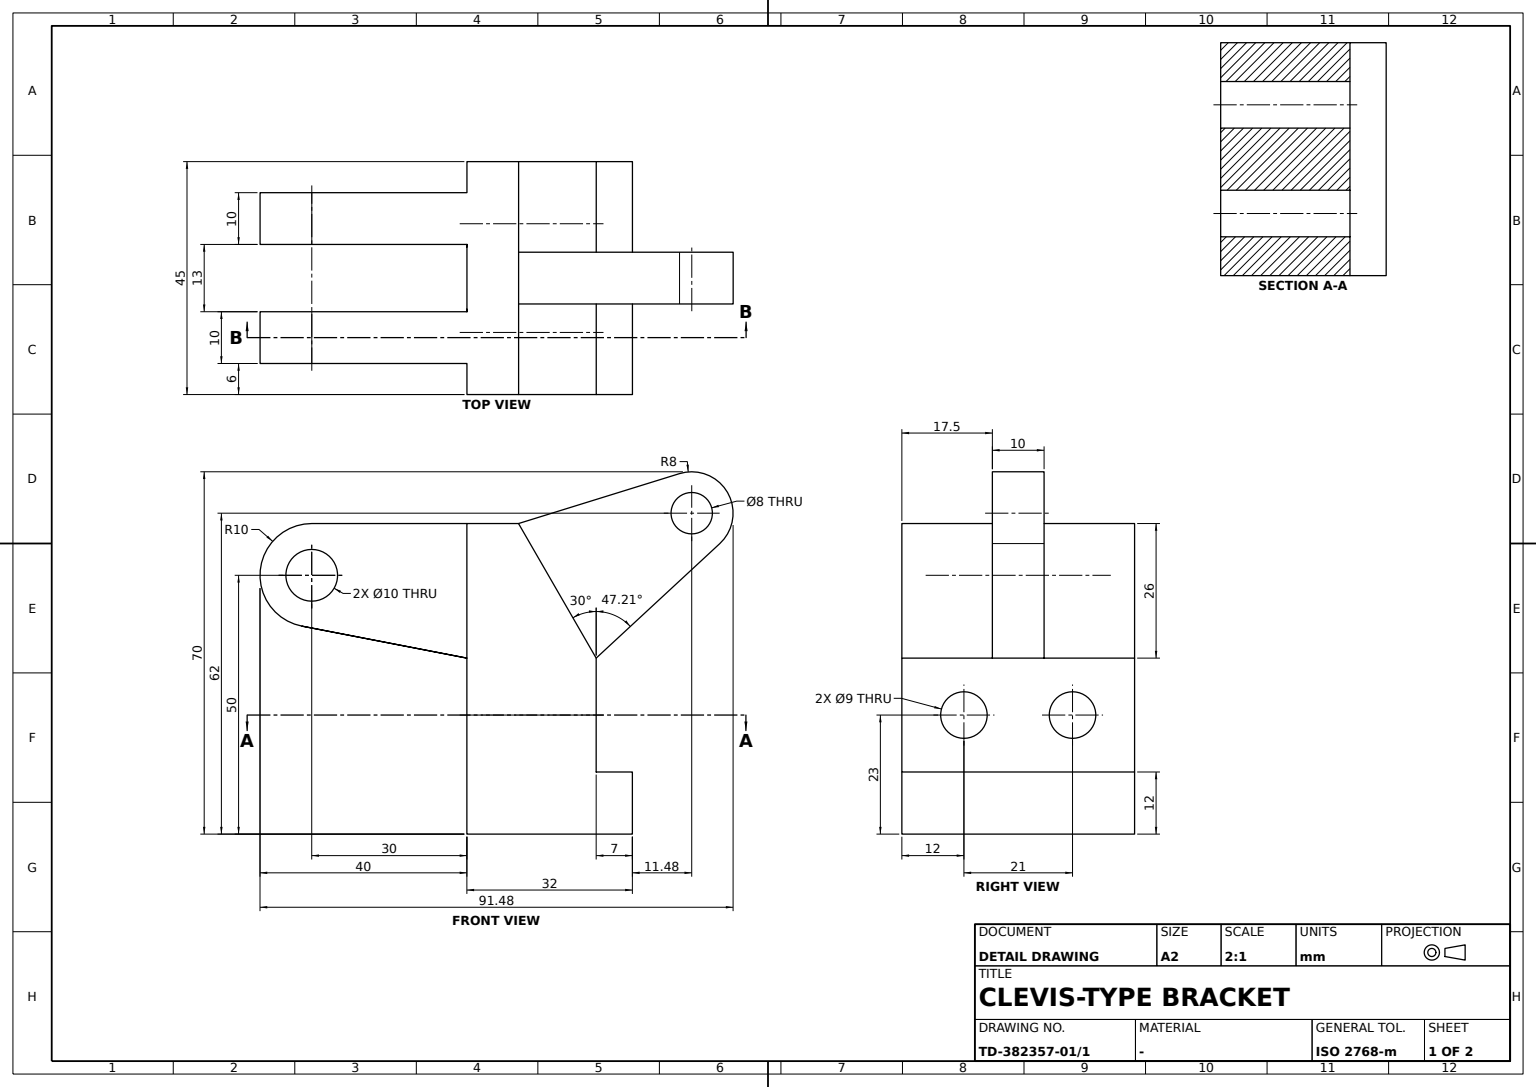
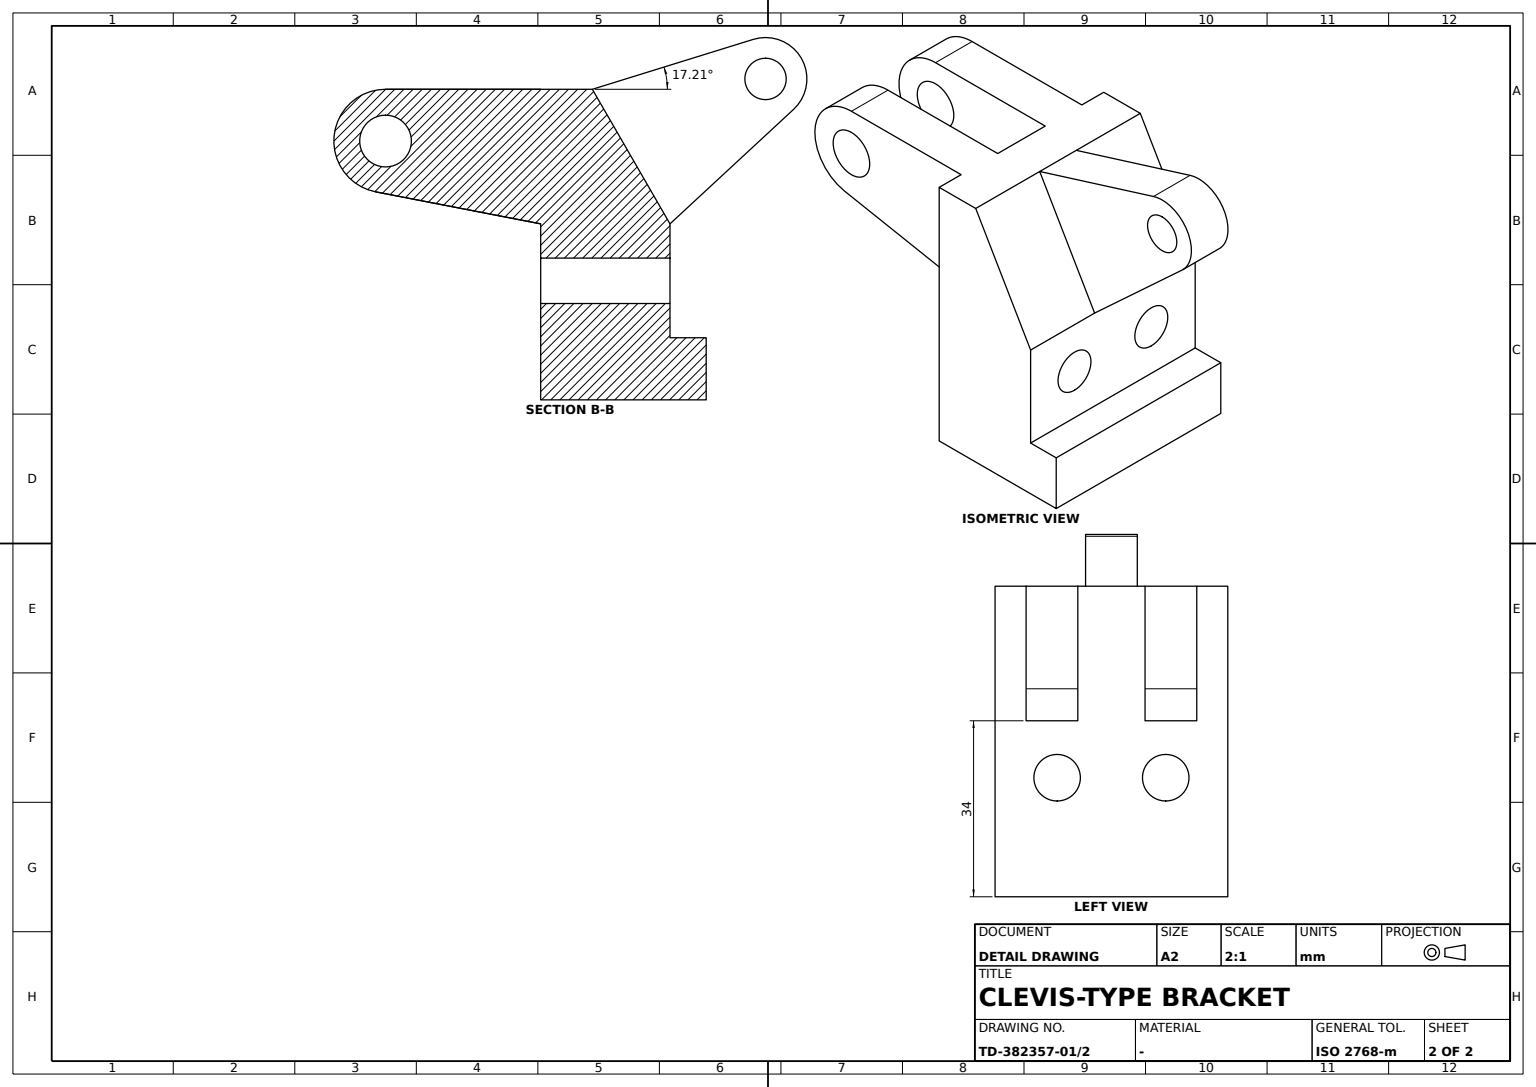
ISO-10303-21;
HEADER;
FILE_DESCRIPTION((''),'2;1');
FILE_NAME('','',(''),(''),'','','');
FILE_SCHEMA(('AUTOMOTIVE_DESIGN'));
ENDSEC;
DATA;
#1=APPLICATION_CONTEXT('');
#2=PRODUCT_CONTEXT('',#1,'mechanical');
#3=PRODUCT('','','',(#2));
#4=PRODUCT_DEFINITION_FORMATION('','',#3);
#5=PRODUCT_DEFINITION_CONTEXT('',#1,'design');
#6=PRODUCT_DEFINITION('','',#4,#5);
#7=PRODUCT_DEFINITION_SHAPE('','',#6);
#8=(LENGTH_UNIT()NAMED_UNIT(*)SI_UNIT(.MILLI.,.METRE.));
#9=(NAMED_UNIT(*)PLANE_ANGLE_UNIT()SI_UNIT($,.RADIAN.));
#10=(NAMED_UNIT(*)SI_UNIT($,.STERADIAN.)SOLID_ANGLE_UNIT());
#11=UNCERTAINTY_MEASURE_WITH_UNIT(LENGTH_MEASURE(0.005),#8,'distance_accuracy_value','');
#12=(GEOMETRIC_REPRESENTATION_CONTEXT(3)GLOBAL_UNCERTAINTY_ASSIGNED_CONTEXT((#11))GLOBAL_UNIT_ASSIGNED_CONTEXT((#8,#9,#10))REPRESENTATION_CONTEXT('',''));
#13=CARTESIAN_POINT('',(0.,22.5,0.));
#14=VERTEX_POINT('',#13);
#15=CARTESIAN_POINT('',(0.,22.5,12.));
#16=VERTEX_POINT('',#15);
#17=DIRECTION('',(0.,0.,1.));
#18=VECTOR('',#17,1000.);
#19=LINE('',#13,#18);
#20=EDGE_CURVE('',#14,#16,#19,.T.);
#21=ORIENTED_EDGE('',*,*,#20,.T.);
#22=CARTESIAN_POINT('',(0.,-22.5,12.));
#23=VERTEX_POINT('',#22);
#24=CARTESIAN_POINT('',(0.,0.,12.));
#25=DIRECTION('',(0.,1.,0.));
#26=VECTOR('',#25,1000.);
#27=LINE('',#24,#26);
#28=EDGE_CURVE('',#23,#16,#27,.T.);
#29=ORIENTED_EDGE('',*,*,#28,.F.);
#30=CARTESIAN_POINT('',(0.,-22.5,0.));
#31=VERTEX_POINT('',#30);
#32=LINE('',#30,#18);
#33=EDGE_CURVE('',#31,#23,#32,.T.);
#34=ORIENTED_EDGE('',*,*,#33,.F.);
#35=CARTESIAN_POINT('',(0.,0.,0.));
#36=LINE('',#35,#26);
#37=EDGE_CURVE('',#31,#14,#36,.T.);
#38=ORIENTED_EDGE('',*,*,#37,.T.);
#39=EDGE_LOOP('',(#21,#29,#34,#38));
#40=FACE_BOUND('',#39,.T.);
#41=DIRECTION('',(-1.,0.,0.));
#42=AXIS2_PLACEMENT_3D('',#35,#41,#17);
#43=PLANE('',#42);
#44=ADVANCED_FACE('',(#40),#43,.F.);
#45=CARTESIAN_POINT('',(-32.,10.5,18.5));
#46=VERTEX_POINT('',#45);
#47=CARTESIAN_POINT('',(-32.,10.5,23.));
#48=DIRECTION('',(1.,0.,0.));
#49=DIRECTION('',(0.,0.,-1.));
#50=AXIS2_PLACEMENT_3D('',#47,#48,#49);
#51=CIRCLE('',#50,4.5);
#52=EDGE_CURVE('',#46,#46,#51,.T.);
#53=ORIENTED_EDGE('',*,*,#52,.T.);
#54=EDGE_LOOP('',(#53));
#55=FACE_BOUND('',#54,.T.);
#56=CARTESIAN_POINT('',(-32.,-16.5,34.));
#57=VERTEX_POINT('',#56);
#58=CARTESIAN_POINT('',(-32.,-6.5,34.));
#59=VERTEX_POINT('',#58);
#60=CARTESIAN_POINT('',(-32.,0.,34.));
#61=LINE('',#60,#26);
#62=EDGE_CURVE('',#57,#59,#61,.T.);
#63=ORIENTED_EDGE('',*,*,#62,.T.);
#64=CARTESIAN_POINT('',(-32.,-6.5,60.));
#65=VERTEX_POINT('',#64);
#66=CARTESIAN_POINT('',(-32.,-6.5,0.));
#67=VECTOR('',#49,1000.);
#68=LINE('',#66,#67);
#69=EDGE_CURVE('',#65,#59,#68,.T.);
#70=ORIENTED_EDGE('',*,*,#69,.F.);
#71=CARTESIAN_POINT('',(-32.,6.5,60.));
#72=VERTEX_POINT('',#71);
#73=CARTESIAN_POINT('',(-32.,0.,60.));
#74=DIRECTION('',(0.,-1.,0.));
#75=VECTOR('',#74,1000.);
#76=LINE('',#73,#75);
#77=EDGE_CURVE('',#65,#72,#76,.F.);
#78=ORIENTED_EDGE('',*,*,#77,.T.);
#79=CARTESIAN_POINT('',(-32.,6.5,34.));
#80=VERTEX_POINT('',#79);
#81=CARTESIAN_POINT('',(-32.,6.5,0.));
#82=LINE('',#81,#67);
#83=EDGE_CURVE('',#72,#80,#82,.T.);
#84=ORIENTED_EDGE('',*,*,#83,.T.);
#85=CARTESIAN_POINT('',(-32.,16.5,34.));
#86=VERTEX_POINT('',#85);
#87=EDGE_CURVE('',#80,#86,#61,.T.);
#88=ORIENTED_EDGE('',*,*,#87,.T.);
#89=CARTESIAN_POINT('',(-32.,16.5,60.));
#90=VERTEX_POINT('',#89);
#91=CARTESIAN_POINT('',(-32.,16.5,0.));
#92=LINE('',#91,#67);
#93=EDGE_CURVE('',#90,#86,#92,.T.);
#94=ORIENTED_EDGE('',*,*,#93,.F.);
#95=CARTESIAN_POINT('',(-32.,22.5,60.));
#96=VERTEX_POINT('',#95);
#97=LINE('',#73,#26);
#98=EDGE_CURVE('',#90,#96,#97,.T.);
#99=ORIENTED_EDGE('',*,*,#98,.T.);
#100=CARTESIAN_POINT('',(-32.,22.5,0.));
#101=VERTEX_POINT('',#100);
#102=LINE('',#100,#67);
#103=EDGE_CURVE('',#96,#101,#102,.T.);
#104=ORIENTED_EDGE('',*,*,#103,.T.);
#105=CARTESIAN_POINT('',(-32.,-22.5,0.));
#106=VERTEX_POINT('',#105);
#107=CARTESIAN_POINT('',(-32.,0.,0.));
#108=LINE('',#107,#26);
#109=EDGE_CURVE('',#106,#101,#108,.T.);
#110=ORIENTED_EDGE('',*,*,#109,.F.);
#111=CARTESIAN_POINT('',(-32.,-22.5,60.));
#112=VERTEX_POINT('',#111);
#113=LINE('',#105,#67);
#114=EDGE_CURVE('',#112,#106,#113,.T.);
#115=ORIENTED_EDGE('',*,*,#114,.F.);
#116=CARTESIAN_POINT('',(-32.,-16.5,60.));
#117=VERTEX_POINT('',#116);
#118=EDGE_CURVE('',#112,#117,#97,.T.);
#119=ORIENTED_EDGE('',*,*,#118,.T.);
#120=CARTESIAN_POINT('',(-32.,-16.5,0.));
#121=LINE('',#120,#67);
#122=EDGE_CURVE('',#117,#57,#121,.T.);
#123=ORIENTED_EDGE('',*,*,#122,.T.);
#124=EDGE_LOOP('',(#63,#70,#78,#84,#88,#94,#99,#104,#110,#115,#119,#123));
#125=FACE_BOUND('',#124,.T.);
#126=CARTESIAN_POINT('',(-32.,-10.5,18.5));
#127=VERTEX_POINT('',#126);
#128=CARTESIAN_POINT('',(-32.,-10.5,23.));
#129=AXIS2_PLACEMENT_3D('',#128,#48,#49);
#130=CIRCLE('',#129,4.5);
#131=EDGE_CURVE('',#127,#127,#130,.T.);
#132=ORIENTED_EDGE('',*,*,#131,.T.);
#133=EDGE_LOOP('',(#132));
#134=FACE_BOUND('',#133,.T.);
#135=AXIS2_PLACEMENT_3D('',#73,#48,#49);
#136=PLANE('',#135);
#137=ADVANCED_FACE('',(#55,#125,#134),#136,.F.);
#138=CARTESIAN_POINT('',(-7.,-5.,34.));
#139=VERTEX_POINT('',#138);
#140=CARTESIAN_POINT('',(16.909194,-5.,56.128873));
#141=VERTEX_POINT('',#140);
#142=CARTESIAN_POINT('',(-20.178941,-5.,21.802386));
#143=DIRECTION('',(0.733902506,0.,0.679254821));
#144=VECTOR('',#143,1000.);
#145=LINE('',#142,#144);
#146=EDGE_CURVE('',#139,#141,#145,.T.);
#147=ORIENTED_EDGE('',*,*,#146,.T.);
#148=CARTESIAN_POINT('',(9.1075,-5.,69.641703));
#149=VERTEX_POINT('',#148);
#150=CARTESIAN_POINT('',(11.475155,-5.,62.000093));
#151=AXIS2_PLACEMENT_3D('',#150,#25,#17);
#152=CIRCLE('',#151,8.);
#153=EDGE_CURVE('',#149,#141,#152,.T.);
#154=ORIENTED_EDGE('',*,*,#153,.F.);
#155=CARTESIAN_POINT('',(-22.011107,-5.,60.));
#156=VERTEX_POINT('',#155);
#157=CARTESIAN_POINT('',(-18.88987,-5.,60.967075));
#158=DIRECTION('',(-0.955201288,0.,-0.295956923));
#159=VECTOR('',#158,1000.);
#160=LINE('',#157,#159);
#161=EDGE_CURVE('',#149,#156,#160,.T.);
#162=ORIENTED_EDGE('',*,*,#161,.T.);
#163=DIRECTION('',(0.5,0.,-0.866025404));
#164=VECTOR('',#163,1000.);
#165=LINE('',#138,#164);
#166=EDGE_CURVE('',#156,#139,#165,.T.);
#167=ORIENTED_EDGE('',*,*,#166,.T.);
#168=EDGE_LOOP('',(#147,#154,#162,#167));
#169=FACE_BOUND('',#168,.T.);
#170=CARTESIAN_POINT('',(11.475155,-5.,66.000093));
#171=VERTEX_POINT('',#170);
#172=CIRCLE('',#151,4.);
#173=EDGE_CURVE('',#171,#171,#172,.T.);
#174=ORIENTED_EDGE('',*,*,#173,.T.);
#175=EDGE_LOOP('',(#174));
#176=FACE_BOUND('',#175,.T.);
#177=CARTESIAN_POINT('',(0.,-5.,0.));
#178=AXIS2_PLACEMENT_3D('',#177,#25,#41);
#179=PLANE('',#178);
#180=ADVANCED_FACE('',(#169,#176),#179,.F.);
#181=ORIENTED_EDGE('',*,*,#87,.F.);
#182=CARTESIAN_POINT('',(-63.902582,6.5,40.182659));
#183=VERTEX_POINT('',#182);
#184=CARTESIAN_POINT('',(5.192278,6.5,26.792208));
#185=DIRECTION('',(-0.98173409,0.,0.190258182));
#186=VECTOR('',#185,1000.);
#187=LINE('',#184,#186);
#188=EDGE_CURVE('',#80,#183,#187,.T.);
#189=ORIENTED_EDGE('',*,*,#188,.T.);
#190=CARTESIAN_POINT('',(-63.902582,16.5,40.182659));
#191=VERTEX_POINT('',#190);
#192=CARTESIAN_POINT('',(-63.902582,0.,40.182659));
#193=LINE('',#192,#26);
#194=EDGE_CURVE('',#183,#191,#193,.T.);
#195=ORIENTED_EDGE('',*,*,#194,.T.);
#196=CARTESIAN_POINT('',(5.192278,16.5,26.792208));
#197=LINE('',#196,#186);
#198=EDGE_CURVE('',#86,#191,#197,.T.);
#199=ORIENTED_EDGE('',*,*,#198,.F.);
#200=EDGE_LOOP('',(#181,#189,#195,#199));
#201=FACE_BOUND('',#200,.T.);
#202=DIRECTION('',(-0.190258182,0.,-0.98173409));
#203=AXIS2_PLACEMENT_3D('',#60,#202,#185);
#204=PLANE('',#203);
#205=ADVANCED_FACE('',(#201),#204,.T.);
#206=CARTESIAN_POINT('',(-62.,16.5,55.));
#207=VERTEX_POINT('',#206);
#208=CARTESIAN_POINT('',(-62.,16.5,50.));
#209=AXIS2_PLACEMENT_3D('',#208,#25,#17);
#210=CIRCLE('',#209,5.);
#211=EDGE_CURVE('',#207,#207,#210,.T.);
#212=ORIENTED_EDGE('',*,*,#211,.T.);
#213=EDGE_LOOP('',(#212));
#214=FACE_BOUND('',#213,.T.);
#215=CARTESIAN_POINT('',(-62.,6.5,55.));
#216=VERTEX_POINT('',#215);
#217=CARTESIAN_POINT('',(-62.,6.5,50.));
#218=AXIS2_PLACEMENT_3D('',#217,#25,#17);
#219=CIRCLE('',#218,5.);
#220=EDGE_CURVE('',#216,#216,#219,.T.);
#221=ORIENTED_EDGE('',*,*,#220,.F.);
#222=EDGE_LOOP('',(#221));
#223=FACE_BOUND('',#222,.T.);
#224=CARTESIAN_POINT('',(-62.,0.,50.));
#225=AXIS2_PLACEMENT_3D('',#224,#25,#41);
#226=CYLINDRICAL_SURFACE('',#225,5.);
#227=ADVANCED_FACE('',(#214,#223),#226,.F.);
#228=ORIENTED_EDGE('',*,*,#28,.T.);
#229=CARTESIAN_POINT('',(-7.,22.5,12.));
#230=VERTEX_POINT('',#229);
#231=VECTOR('',#41,1000.);
#232=LINE('',#15,#231);
#233=EDGE_CURVE('',#16,#230,#232,.T.);
#234=ORIENTED_EDGE('',*,*,#233,.T.);
#235=CARTESIAN_POINT('',(-7.,-22.5,12.));
#236=VERTEX_POINT('',#235);
#237=CARTESIAN_POINT('',(-7.,0.,12.));
#238=LINE('',#237,#26);
#239=EDGE_CURVE('',#236,#230,#238,.T.);
#240=ORIENTED_EDGE('',*,*,#239,.F.);
#241=LINE('',#22,#231);
#242=EDGE_CURVE('',#23,#236,#241,.T.);
#243=ORIENTED_EDGE('',*,*,#242,.F.);
#244=EDGE_LOOP('',(#228,#234,#240,#243));
#245=FACE_BOUND('',#244,.T.);
#246=AXIS2_PLACEMENT_3D('',#24,#49,#41);
#247=PLANE('',#246);
#248=ADVANCED_FACE('',(#245),#247,.F.);
#249=ORIENTED_EDGE('',*,*,#77,.F.);
#250=CARTESIAN_POINT('',(-62.,-6.5,60.));
#251=VERTEX_POINT('',#250);
#252=CARTESIAN_POINT('',(-22.011107,-6.5,60.));
#253=VECTOR('',#48,1000.);
#254=LINE('',#252,#253);
#255=EDGE_CURVE('',#251,#65,#254,.T.);
#256=ORIENTED_EDGE('',*,*,#255,.F.);
#257=CARTESIAN_POINT('',(-62.,-16.5,60.));
#258=VERTEX_POINT('',#257);
#259=CARTESIAN_POINT('',(-62.,0.,60.));
#260=LINE('',#259,#26);
#261=EDGE_CURVE('',#258,#251,#260,.T.);
#262=ORIENTED_EDGE('',*,*,#261,.F.);
#263=CARTESIAN_POINT('',(0.,-16.5,60.));
#264=LINE('',#263,#231);
#265=EDGE_CURVE('',#117,#258,#264,.T.);
#266=ORIENTED_EDGE('',*,*,#265,.F.);
#267=ORIENTED_EDGE('',*,*,#118,.F.);
#268=CARTESIAN_POINT('',(-22.011107,-22.5,60.));
#269=VERTEX_POINT('',#268);
#270=CARTESIAN_POINT('',(0.,-22.5,60.));
#271=LINE('',#270,#231);
#272=EDGE_CURVE('',#269,#112,#271,.T.);
#273=ORIENTED_EDGE('',*,*,#272,.F.);
#274=CARTESIAN_POINT('',(-22.011107,0.,60.));
#275=LINE('',#274,#26);
#276=EDGE_CURVE('',#269,#156,#275,.T.);
#277=ORIENTED_EDGE('',*,*,#276,.T.);
#278=CARTESIAN_POINT('',(-22.011107,5.,60.));
#279=VERTEX_POINT('',#278);
#280=EDGE_CURVE('',#156,#279,#275,.T.);
#281=ORIENTED_EDGE('',*,*,#280,.T.);
#282=CARTESIAN_POINT('',(-22.011107,22.5,60.));
#283=VERTEX_POINT('',#282);
#284=EDGE_CURVE('',#279,#283,#275,.T.);
#285=ORIENTED_EDGE('',*,*,#284,.T.);
#286=CARTESIAN_POINT('',(0.,22.5,60.));
#287=LINE('',#286,#231);
#288=EDGE_CURVE('',#283,#96,#287,.T.);
#289=ORIENTED_EDGE('',*,*,#288,.T.);
#290=ORIENTED_EDGE('',*,*,#98,.F.);
#291=CARTESIAN_POINT('',(-62.,16.5,60.));
#292=VERTEX_POINT('',#291);
#293=CARTESIAN_POINT('',(0.,16.5,60.));
#294=LINE('',#293,#231);
#295=EDGE_CURVE('',#90,#292,#294,.T.);
#296=ORIENTED_EDGE('',*,*,#295,.T.);
#297=CARTESIAN_POINT('',(-62.,6.5,60.));
#298=VERTEX_POINT('',#297);
#299=EDGE_CURVE('',#298,#292,#260,.T.);
#300=ORIENTED_EDGE('',*,*,#299,.F.);
#301=CARTESIAN_POINT('',(-22.011107,6.5,60.));
#302=LINE('',#301,#253);
#303=EDGE_CURVE('',#298,#72,#302,.T.);
#304=ORIENTED_EDGE('',*,*,#303,.T.);
#305=EDGE_LOOP('',(#249,#256,#262,#266,#267,#273,#277,#281,#285,#289,#290,#296,#300,#304));
#306=FACE_BOUND('',#305,.T.);
#307=AXIS2_PLACEMENT_3D('',#274,#49,#41);
#308=PLANE('',#307);
#309=ADVANCED_FACE('',(#306),#308,.F.);
#310=CARTESIAN_POINT('',(-63.902582,-6.5,40.182659));
#311=VERTEX_POINT('',#310);
#312=CARTESIAN_POINT('',(5.192278,-6.5,26.792208));
#313=LINE('',#312,#186);
#314=EDGE_CURVE('',#59,#311,#313,.T.);
#315=ORIENTED_EDGE('',*,*,#314,.F.);
#316=ORIENTED_EDGE('',*,*,#62,.F.);
#317=CARTESIAN_POINT('',(-63.902582,-16.5,40.182659));
#318=VERTEX_POINT('',#317);
#319=CARTESIAN_POINT('',(5.192278,-16.5,26.792208));
#320=LINE('',#319,#186);
#321=EDGE_CURVE('',#57,#318,#320,.T.);
#322=ORIENTED_EDGE('',*,*,#321,.T.);
#323=EDGE_CURVE('',#318,#311,#193,.T.);
#324=ORIENTED_EDGE('',*,*,#323,.T.);
#325=EDGE_LOOP('',(#315,#316,#322,#324));
#326=FACE_BOUND('',#325,.T.);
#327=ADVANCED_FACE('',(#326),#204,.T.);
#328=ORIENTED_EDGE('',*,*,#323,.F.);
#329=CARTESIAN_POINT('',(-62.,-16.5,50.));
#330=AXIS2_PLACEMENT_3D('',#329,#25,#17);
#331=CIRCLE('',#330,10.);
#332=EDGE_CURVE('',#318,#258,#331,.T.);
#333=ORIENTED_EDGE('',*,*,#332,.T.);
#334=ORIENTED_EDGE('',*,*,#261,.T.);
#335=CARTESIAN_POINT('',(-62.,-6.5,50.));
#336=AXIS2_PLACEMENT_3D('',#335,#25,#17);
#337=CIRCLE('',#336,10.);
#338=EDGE_CURVE('',#311,#251,#337,.T.);
#339=ORIENTED_EDGE('',*,*,#338,.F.);
#340=EDGE_LOOP('',(#328,#333,#334,#339));
#341=FACE_BOUND('',#340,.T.);
#342=CYLINDRICAL_SURFACE('',#225,10.);
#343=ADVANCED_FACE('',(#341),#342,.T.);
#344=CARTESIAN_POINT('',(-7.,22.5,34.));
#345=VERTEX_POINT('',#344);
#346=CARTESIAN_POINT('',(-7.,22.5,0.));
#347=LINE('',#346,#18);
#348=EDGE_CURVE('',#230,#345,#347,.T.);
#349=ORIENTED_EDGE('',*,*,#348,.F.);
#350=ORIENTED_EDGE('',*,*,#233,.F.);
#351=ORIENTED_EDGE('',*,*,#20,.F.);
#352=LINE('',#13,#253);
#353=EDGE_CURVE('',#101,#14,#352,.T.);
#354=ORIENTED_EDGE('',*,*,#353,.F.);
#355=ORIENTED_EDGE('',*,*,#103,.F.);
#356=ORIENTED_EDGE('',*,*,#288,.F.);
#357=CARTESIAN_POINT('',(9.472432,22.5,5.468911));
#358=DIRECTION('',(-0.5,0.,0.866025404));
#359=VECTOR('',#358,1000.);
#360=LINE('',#357,#359);
#361=EDGE_CURVE('',#345,#283,#360,.T.);
#362=ORIENTED_EDGE('',*,*,#361,.F.);
#363=EDGE_LOOP('',(#349,#350,#351,#354,#355,#356,#362));
#364=FACE_BOUND('',#363,.T.);
#365=AXIS2_PLACEMENT_3D('',#13,#25,#41);
#366=PLANE('',#365);
#367=ADVANCED_FACE('',(#364),#366,.T.);
#368=CARTESIAN_POINT('',(-7.,-10.5,27.5));
#369=VERTEX_POINT('',#368);
#370=CARTESIAN_POINT('',(-7.,-10.5,23.));
#371=AXIS2_PLACEMENT_3D('',#370,#41,#17);
#372=CIRCLE('',#371,4.5);
#373=EDGE_CURVE('',#369,#369,#372,.T.);
#374=ORIENTED_EDGE('',*,*,#373,.F.);
#375=EDGE_LOOP('',(#374));
#376=FACE_BOUND('',#375,.T.);
#377=ORIENTED_EDGE('',*,*,#131,.F.);
#378=EDGE_LOOP('',(#377));
#379=FACE_BOUND('',#378,.T.);
#380=CARTESIAN_POINT('',(-20.,-10.5,23.));
#381=AXIS2_PLACEMENT_3D('',#380,#48,#25);
#382=CYLINDRICAL_SURFACE('',#381,4.5);
#383=ADVANCED_FACE('',(#376,#379),#382,.F.);
#384=CARTESIAN_POINT('',(-7.,10.5,27.5));
#385=VERTEX_POINT('',#384);
#386=CARTESIAN_POINT('',(-7.,10.5,23.));
#387=AXIS2_PLACEMENT_3D('',#386,#41,#17);
#388=CIRCLE('',#387,4.5);
#389=EDGE_CURVE('',#385,#385,#388,.T.);
#390=ORIENTED_EDGE('',*,*,#389,.T.);
#391=EDGE_LOOP('',(#390));
#392=FACE_BOUND('',#391,.T.);
#393=CARTESIAN_POINT('',(-7.,5.,34.));
#394=VERTEX_POINT('',#393);
#395=CARTESIAN_POINT('',(-7.,0.,34.));
#396=LINE('',#395,#26);
#397=EDGE_CURVE('',#394,#345,#396,.T.);
#398=ORIENTED_EDGE('',*,*,#397,.F.);
#399=EDGE_CURVE('',#139,#394,#396,.T.);
#400=ORIENTED_EDGE('',*,*,#399,.F.);
#401=CARTESIAN_POINT('',(-7.,-22.5,34.));
#402=VERTEX_POINT('',#401);
#403=EDGE_CURVE('',#402,#139,#396,.T.);
#404=ORIENTED_EDGE('',*,*,#403,.F.);
#405=CARTESIAN_POINT('',(-7.,-22.5,0.));
#406=LINE('',#405,#18);
#407=EDGE_CURVE('',#236,#402,#406,.T.);
#408=ORIENTED_EDGE('',*,*,#407,.F.);
#409=ORIENTED_EDGE('',*,*,#239,.T.);
#410=ORIENTED_EDGE('',*,*,#348,.T.);
#411=EDGE_LOOP('',(#398,#400,#404,#408,#409,#410));
#412=FACE_BOUND('',#411,.T.);
#413=ORIENTED_EDGE('',*,*,#373,.T.);
#414=EDGE_LOOP('',(#413));
#415=FACE_BOUND('',#414,.T.);
#416=AXIS2_PLACEMENT_3D('',#237,#41,#17);
#417=PLANE('',#416);
#418=ADVANCED_FACE('',(#392,#412,#415),#417,.F.);
#419=ORIENTED_EDGE('',*,*,#389,.F.);
#420=EDGE_LOOP('',(#419));
#421=FACE_BOUND('',#420,.T.);
#422=ORIENTED_EDGE('',*,*,#52,.F.);
#423=EDGE_LOOP('',(#422));
#424=FACE_BOUND('',#423,.T.);
#425=CARTESIAN_POINT('',(-20.,10.5,23.));
#426=AXIS2_PLACEMENT_3D('',#425,#48,#25);
#427=CYLINDRICAL_SURFACE('',#426,4.5);
#428=ADVANCED_FACE('',(#421,#424),#427,.F.);
#429=ORIENTED_EDGE('',*,*,#361,.T.);
#430=ORIENTED_EDGE('',*,*,#284,.F.);
#431=LINE('',#393,#164);
#432=EDGE_CURVE('',#279,#394,#431,.T.);
#433=ORIENTED_EDGE('',*,*,#432,.T.);
#434=ORIENTED_EDGE('',*,*,#397,.T.);
#435=EDGE_LOOP('',(#429,#430,#433,#434));
#436=FACE_BOUND('',#435,.T.);
#437=DIRECTION('',(-0.866025404,0.,-0.5));
#438=AXIS2_PLACEMENT_3D('',#395,#437,#358);
#439=PLANE('',#438);
#440=ADVANCED_FACE('',(#436),#439,.F.);
#441=CARTESIAN_POINT('',(-62.,-6.5,55.));
#442=VERTEX_POINT('',#441);
#443=CIRCLE('',#336,5.);
#444=EDGE_CURVE('',#442,#442,#443,.T.);
#445=ORIENTED_EDGE('',*,*,#444,.T.);
#446=EDGE_LOOP('',(#445));
#447=FACE_BOUND('',#446,.T.);
#448=CARTESIAN_POINT('',(-62.,-16.5,55.));
#449=VERTEX_POINT('',#448);
#450=CIRCLE('',#330,5.);
#451=EDGE_CURVE('',#449,#449,#450,.T.);
#452=ORIENTED_EDGE('',*,*,#451,.F.);
#453=EDGE_LOOP('',(#452));
#454=FACE_BOUND('',#453,.T.);
#455=ADVANCED_FACE('',(#447,#454),#226,.F.);
#456=CARTESIAN_POINT('',(16.909194,5.,56.128873));
#457=VERTEX_POINT('',#456);
#458=CARTESIAN_POINT('',(-20.178941,5.,21.802386));
#459=LINE('',#458,#144);
#460=EDGE_CURVE('',#394,#457,#459,.T.);
#461=ORIENTED_EDGE('',*,*,#460,.T.);
#462=CARTESIAN_POINT('',(16.909194,0.,56.128873));
#463=LINE('',#462,#26);
#464=EDGE_CURVE('',#141,#457,#463,.T.);
#465=ORIENTED_EDGE('',*,*,#464,.F.);
#466=ORIENTED_EDGE('',*,*,#146,.F.);
#467=ORIENTED_EDGE('',*,*,#399,.T.);
#468=EDGE_LOOP('',(#461,#465,#466,#467));
#469=FACE_BOUND('',#468,.T.);
#470=DIRECTION('',(-0.679254821,0.,0.733902506));
#471=AXIS2_PLACEMENT_3D('',#395,#470,#143);
#472=PLANE('',#471);
#473=ADVANCED_FACE('',(#469),#472,.F.);
#474=ORIENTED_EDGE('',*,*,#255,.T.);
#475=ORIENTED_EDGE('',*,*,#69,.T.);
#476=ORIENTED_EDGE('',*,*,#314,.T.);
#477=ORIENTED_EDGE('',*,*,#338,.T.);
#478=EDGE_LOOP('',(#474,#475,#476,#477));
#479=FACE_BOUND('',#478,.T.);
#480=ORIENTED_EDGE('',*,*,#444,.F.);
#481=EDGE_LOOP('',(#480));
#482=FACE_BOUND('',#481,.T.);
#483=CARTESIAN_POINT('',(0.,-6.5,0.));
#484=AXIS2_PLACEMENT_3D('',#483,#25,#41);
#485=PLANE('',#484);
#486=ADVANCED_FACE('',(#479,#482),#485,.T.);
#487=ORIENTED_EDGE('',*,*,#299,.T.);
#488=CIRCLE('',#209,10.);
#489=EDGE_CURVE('',#191,#292,#488,.T.);
#490=ORIENTED_EDGE('',*,*,#489,.F.);
#491=ORIENTED_EDGE('',*,*,#194,.F.);
#492=CIRCLE('',#218,10.);
#493=EDGE_CURVE('',#183,#298,#492,.T.);
#494=ORIENTED_EDGE('',*,*,#493,.T.);
#495=EDGE_LOOP('',(#487,#490,#491,#494));
#496=FACE_BOUND('',#495,.T.);
#497=ADVANCED_FACE('',(#496),#342,.T.);
#498=ORIENTED_EDGE('',*,*,#353,.T.);
#499=ORIENTED_EDGE('',*,*,#37,.F.);
#500=LINE('',#30,#253);
#501=EDGE_CURVE('',#106,#31,#500,.T.);
#502=ORIENTED_EDGE('',*,*,#501,.F.);
#503=ORIENTED_EDGE('',*,*,#109,.T.);
#504=EDGE_LOOP('',(#498,#499,#502,#503));
#505=FACE_BOUND('',#504,.T.);
#506=AXIS2_PLACEMENT_3D('',#107,#17,#48);
#507=PLANE('',#506);
#508=ADVANCED_FACE('',(#505),#507,.F.);
#509=CARTESIAN_POINT('',(9.1075,5.,69.641703));
#510=VERTEX_POINT('',#509);
#511=CARTESIAN_POINT('',(-18.88987,5.,60.967075));
#512=LINE('',#511,#159);
#513=EDGE_CURVE('',#510,#279,#512,.T.);
#514=ORIENTED_EDGE('',*,*,#513,.T.);
#515=ORIENTED_EDGE('',*,*,#280,.F.);
#516=ORIENTED_EDGE('',*,*,#161,.F.);
#517=CARTESIAN_POINT('',(9.1075,0.,69.641703));
#518=LINE('',#517,#26);
#519=EDGE_CURVE('',#149,#510,#518,.T.);
#520=ORIENTED_EDGE('',*,*,#519,.T.);
#521=EDGE_LOOP('',(#514,#515,#516,#520));
#522=FACE_BOUND('',#521,.T.);
#523=DIRECTION('',(0.295956923,0.,-0.955201288));
#524=AXIS2_PLACEMENT_3D('',#517,#523,#158);
#525=PLANE('',#524);
#526=ADVANCED_FACE('',(#522),#525,.F.);
#527=ORIENTED_EDGE('',*,*,#451,.T.);
#528=EDGE_LOOP('',(#527));
#529=FACE_BOUND('',#528,.T.);
#530=ORIENTED_EDGE('',*,*,#321,.F.);
#531=ORIENTED_EDGE('',*,*,#122,.F.);
#532=ORIENTED_EDGE('',*,*,#265,.T.);
#533=ORIENTED_EDGE('',*,*,#332,.F.);
#534=EDGE_LOOP('',(#530,#531,#532,#533));
#535=FACE_BOUND('',#534,.T.);
#536=CARTESIAN_POINT('',(0.,-16.5,0.));
#537=AXIS2_PLACEMENT_3D('',#536,#25,#41);
#538=PLANE('',#537);
#539=ADVANCED_FACE('',(#529,#535),#538,.F.);
#540=CARTESIAN_POINT('',(11.475155,5.,62.000093));
#541=AXIS2_PLACEMENT_3D('',#540,#25,#17);
#542=CIRCLE('',#541,8.);
#543=EDGE_CURVE('',#510,#457,#542,.T.);
#544=ORIENTED_EDGE('',*,*,#543,.F.);
#545=ORIENTED_EDGE('',*,*,#519,.F.);
#546=ORIENTED_EDGE('',*,*,#153,.T.);
#547=ORIENTED_EDGE('',*,*,#464,.T.);
#548=EDGE_LOOP('',(#544,#545,#546,#547));
#549=FACE_BOUND('',#548,.T.);
#550=CARTESIAN_POINT('',(11.475155,0.,62.000093));
#551=AXIS2_PLACEMENT_3D('',#550,#25,#41);
#552=CYLINDRICAL_SURFACE('',#551,8.);
#553=ADVANCED_FACE('',(#549),#552,.T.);
#554=ORIENTED_EDGE('',*,*,#276,.F.);
#555=CARTESIAN_POINT('',(9.472432,-22.5,5.468911));
#556=LINE('',#555,#359);
#557=EDGE_CURVE('',#402,#269,#556,.T.);
#558=ORIENTED_EDGE('',*,*,#557,.F.);
#559=ORIENTED_EDGE('',*,*,#403,.T.);
#560=ORIENTED_EDGE('',*,*,#166,.F.);
#561=EDGE_LOOP('',(#554,#558,#559,#560));
#562=FACE_BOUND('',#561,.T.);
#563=ADVANCED_FACE('',(#562),#439,.F.);
#564=ORIENTED_EDGE('',*,*,#220,.T.);
#565=EDGE_LOOP('',(#564));
#566=FACE_BOUND('',#565,.T.);
#567=ORIENTED_EDGE('',*,*,#83,.F.);
#568=ORIENTED_EDGE('',*,*,#303,.F.);
#569=ORIENTED_EDGE('',*,*,#493,.F.);
#570=ORIENTED_EDGE('',*,*,#188,.F.);
#571=EDGE_LOOP('',(#567,#568,#569,#570));
#572=FACE_BOUND('',#571,.T.);
#573=CARTESIAN_POINT('',(0.,6.5,0.));
#574=AXIS2_PLACEMENT_3D('',#573,#25,#41);
#575=PLANE('',#574);
#576=ADVANCED_FACE('',(#566,#572),#575,.F.);
#577=ORIENTED_EDGE('',*,*,#432,.F.);
#578=ORIENTED_EDGE('',*,*,#513,.F.);
#579=ORIENTED_EDGE('',*,*,#543,.T.);
#580=ORIENTED_EDGE('',*,*,#460,.F.);
#581=EDGE_LOOP('',(#577,#578,#579,#580));
#582=FACE_BOUND('',#581,.T.);
#583=CARTESIAN_POINT('',(11.475155,5.,66.000093));
#584=VERTEX_POINT('',#583);
#585=CIRCLE('',#541,4.);
#586=EDGE_CURVE('',#584,#584,#585,.T.);
#587=ORIENTED_EDGE('',*,*,#586,.F.);
#588=EDGE_LOOP('',(#587));
#589=FACE_BOUND('',#588,.T.);
#590=CARTESIAN_POINT('',(0.,5.,0.));
#591=AXIS2_PLACEMENT_3D('',#590,#25,#41);
#592=PLANE('',#591);
#593=ADVANCED_FACE('',(#582,#589),#592,.T.);
#594=ORIENTED_EDGE('',*,*,#501,.T.);
#595=ORIENTED_EDGE('',*,*,#33,.T.);
#596=ORIENTED_EDGE('',*,*,#242,.T.);
#597=ORIENTED_EDGE('',*,*,#407,.T.);
#598=ORIENTED_EDGE('',*,*,#557,.T.);
#599=ORIENTED_EDGE('',*,*,#272,.T.);
#600=ORIENTED_EDGE('',*,*,#114,.T.);
#601=EDGE_LOOP('',(#594,#595,#596,#597,#598,#599,#600));
#602=FACE_BOUND('',#601,.T.);
#603=AXIS2_PLACEMENT_3D('',#30,#25,#41);
#604=PLANE('',#603);
#605=ADVANCED_FACE('',(#602),#604,.F.);
#606=ORIENTED_EDGE('',*,*,#211,.F.);
#607=EDGE_LOOP('',(#606));
#608=FACE_BOUND('',#607,.T.);
#609=ORIENTED_EDGE('',*,*,#198,.T.);
#610=ORIENTED_EDGE('',*,*,#489,.T.);
#611=ORIENTED_EDGE('',*,*,#295,.F.);
#612=ORIENTED_EDGE('',*,*,#93,.T.);
#613=EDGE_LOOP('',(#609,#610,#611,#612));
#614=FACE_BOUND('',#613,.T.);
#615=CARTESIAN_POINT('',(0.,16.5,0.));
#616=AXIS2_PLACEMENT_3D('',#615,#25,#41);
#617=PLANE('',#616);
#618=ADVANCED_FACE('',(#608,#614),#617,.T.);
#619=ORIENTED_EDGE('',*,*,#586,.T.);
#620=EDGE_LOOP('',(#619));
#621=FACE_BOUND('',#620,.T.);
#622=ORIENTED_EDGE('',*,*,#173,.F.);
#623=EDGE_LOOP('',(#622));
#624=FACE_BOUND('',#623,.T.);
#625=CYLINDRICAL_SURFACE('',#551,4.);
#626=ADVANCED_FACE('',(#621,#624),#625,.F.);
#627=CLOSED_SHELL('',(#44,#137,#180,#205,#227,#248,#309,#327,#343,#367,#383,#418,#428,#440,#455,#473,#486,#497,#508,#526,#539,#553,#563,#576,#593,#605,#618,#626));
#628=MANIFOLD_SOLID_BREP('',#627);
#629=ADVANCED_BREP_SHAPE_REPRESENTATION('',(#628),#12);
#630=SHAPE_DEFINITION_REPRESENTATION(#7,#629);
ENDSEC;
END-ISO-10303-21;
